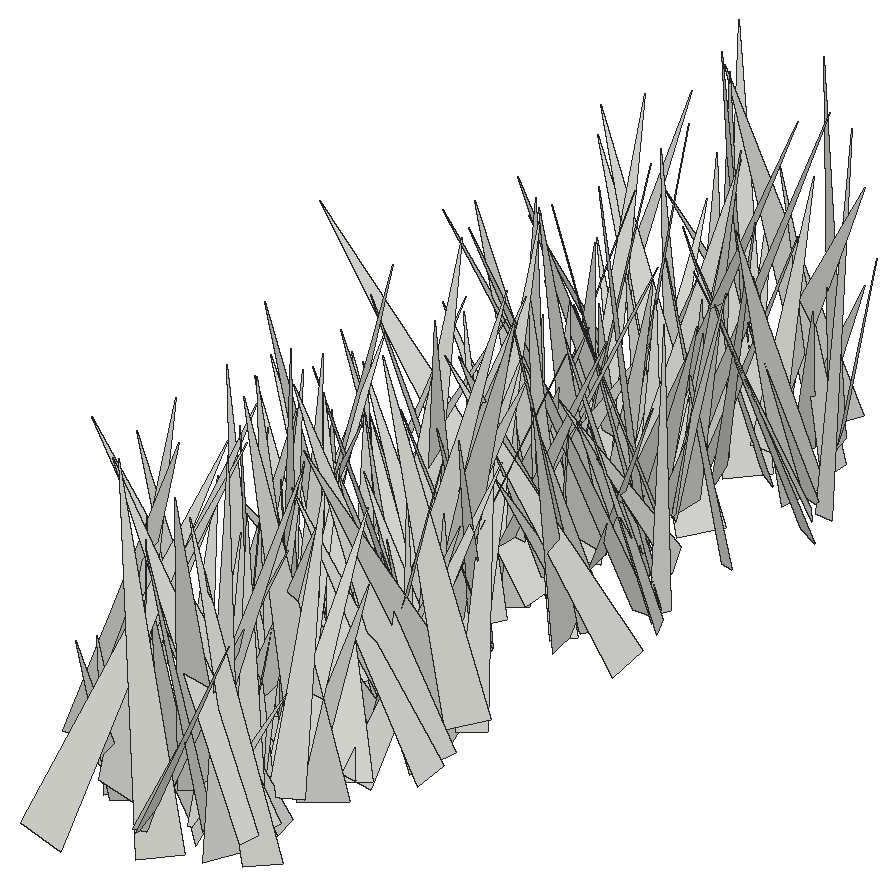
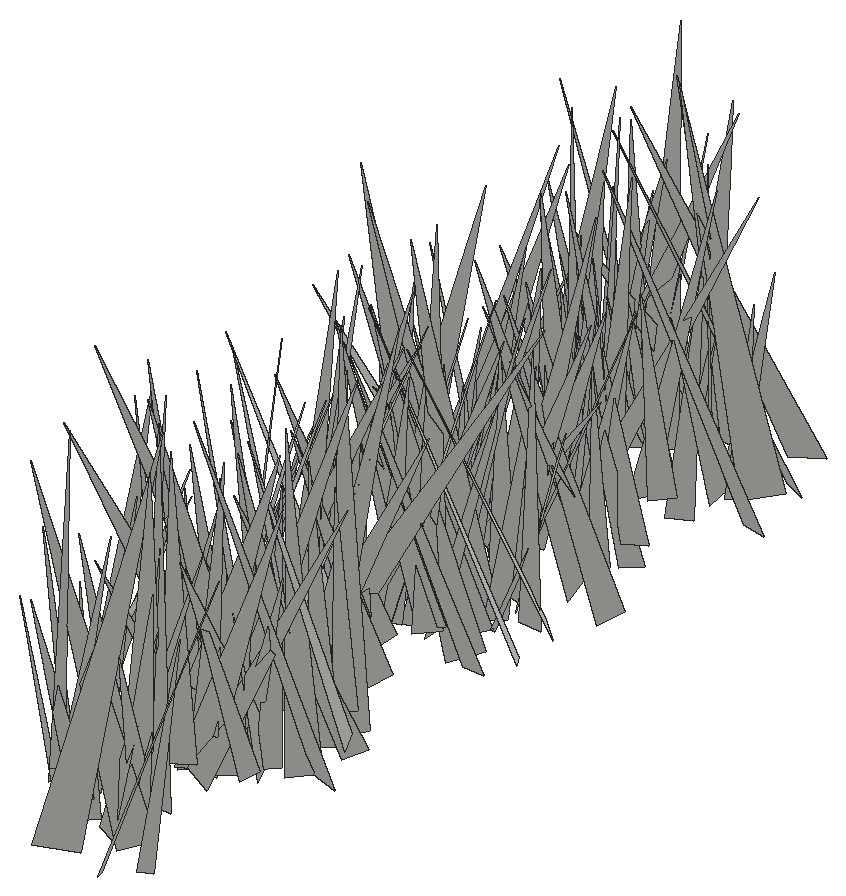
# SketchUp Ruby script. Lengths in inches.
U = 1.inch
M = Sketchup.active_model
def pt(a) = Geom::Point3d.new(a.map { |v| v * U })
def face(e, loops, mat)
  f = e.add_face(loops[0].map { |a| pt(a) })
  loops[1..].each { |l| e.add_face(l.map { |a| pt(a) }).erase! }
  f.material = f.back_material = mat if mat
  f
end
# faces: each face lists its corners as indices into pts; further lists are holes
def faces(e, pts, list, mat = nil) = list.each { |f| face(e, (f[0].is_a?(Array) ? f : [f]).map { |l| l.map { |i| pts[i] } }, mat) }
# xy, xz, yz: faces in a plane at the given z, y or x. An outline is a flat list of corners, or four numbers for a rectangle; further outlines are holes
def ring(l) = l.size == 4 ? [[l[0], l[1]], [l[2], l[1]], [l[2], l[3]], [l[0], l[3]]] : l.each_slice(2).to_a
def flat(e, list, mat, &to3) = list.each { |f| face(e, (f[0].is_a?(Array) ? f : [f]).map { |l| ring(l).map { |u, v| to3.(u, v) } }, mat) }
def xy(e, z, list, mat = nil) = flat(e, list, mat) { |x, y| [x, y, z] }
def xz(e, y, list, mat = nil) = flat(e, list, mat) { |x, z| [x, y, z] }
def yz(e, x, list, mat = nil) = flat(e, list, mat) { |y, z| [x, y, z] }
def lines(e, pts, list) = list.each { |a, b| e.add_line(pt(pts[a]), pt(pts[b])) }
# prism: a flat outline (further loops are holes) pulled along v
def prism(e, loops, v, mat = nil)
  f = face(e, loops, mat); d = Geom::Vector3d.new(v.map { |x| x * U })
  f.pushpull(f.normal.samedirection?(d) ? d.length : -d.length)
end
def box(e, o, s, mat = nil) = prism(e, [[o, [o[0] + s[0], o[1], o[2]], [o[0] + s[0], o[1] + s[1], o[2]], [o[0], o[1] + s[1], o[2]]]], [0, 0, s[2]], mat)
def at(x, y, z, deg = 0) = Geom::Transformation.translation(pt([x, y, z])) * Geom::Transformation.rotation(ORIGIN, Z_AXIS, deg.degrees)
def axes(o, x, y, z) = Geom::Transformation.new([*x, 0, *y, 0, *z, 0, *pt(o).to_a, 1])
def part(name) = M.definitions.add(name)
# library, detail: a bought-in or finely detailed component or shape, given as its bounding box
def library(name, o, s) = part(name).tap { |d| box(d.entities, o, s) }
def detail(e, o, s) = box(e.add_group.entities, o, s)
def put(e, d, t, mat = nil) = e.add_instance(d, t).tap { |i| i.material = mat if mat }
def group(e, t, mat = nil) = e.add_group.tap { |g| g.transformation = t; g.material = mat if mat }.entities
root = M.entities
c1 = part("fur_instance\#9")
p = [[0.8125,0,1.79],[0.67,-0.02,1.48],[0,-0.11,0],[0,0.11,0]]
faces(c1.entities,p,[[0,1,2,3]])
put(root,c1,axes([151.81,72.7,-28.22],[-5.03128,5.10175,2.45438],[5.52933,5.13327,0.66454],[1.21582,-2.23324,7.13442]))
put(root,c1,axes([151.36,72.26,-27.1],[3.9948,0.59542,0.26899],[0.55235,-3.96784,0.58004],[-0.34899,0.53573,3.99706]))
put(root,c1,axes([152.68,74.1,-27.1],[-4.88015,-2.78524,1.52655],[-2.68194,5.11285,0.7548],[1.7015,0.07051,5.5681]))
put(root,c1,axes([151.31,75.63,-27.1],[4.3126,-6.65441,0.44802],[-6.65528,-4.32849,-0.22777],[-0.435,0.25174,7.9264]))
put(root,c1,axes([148.35,74.96,-28.22],[1.6071,-3.85332,0.26864],[-3.82652,-1.62792,-0.45895],[-0.52725,0.06941,4.14972]))
put(root,c1,axes([147.79,71.21,-28.22],[0.28527,8.21503,1.11931],[7.94931,0.04717,-2.37217],[2.35543,-1.15413,7.87026]))
put(root,c1,axes([154.69,74.52,-27.1],[-6.88709,2.46248,0.81316],[2.58785,6.67518,1.70354],[0.16756,-1.88022,7.11293]))
put(root,c1,axes([151.44,73.41,-28.22],[1.87721,3.55983,2.07479],[3.45548,-2.60202,1.33802],[-2.2443,-1.02868,3.79553]))
put(root,c1,axes([149.46,74.71,-27.1],[4.52719,2.71843,2.25301],[3.1828,-4.72799,-0.69084],[-1.52829,-1.79378,5.23527]))
put(root,c1,axes([147.89,75.2,-28.22],[2.32734,-2.83374,0.7234],[-2.82694,-2.41664,-0.37171],[-0.74954,0.31569,3.64807]))
put(root,c1,axes([154.875,74.43,-28.22],[1.40362,-5.52471,3.15038],[-5.88186,-2.35471,-1.50878],[-2.41887,2.51999,5.49692]))
put(root,c1,axes([149.01,73.77,-27.1],[1.36969,7.27883,2.41401],[7.66649,-1.2409,-0.6083],[0.18385,-2.48268,7.38156]))
put(root,c1,axes([146.77,74.74,-27.1],[4.56446,-0.76979,0.5853],[-0.81155,-4.58493,0.29877],[-0.52586,0.39409,4.61927]))
put(root,c1,axes([153.43,73.97,-28.22],[-6.82221,1.72842,2.33339],[1.55801,7.20655,-0.7829],[2.45045,0.23004,6.99407]))
put(root,c1,axes([146,76,-27.1],[4.04324,-6.81137,0.9787],[-6.74817,-3.70246,2.11055],[1.34718,1.89668,7.63467]))
put(root,c1,axes([151.84,74.47,-28.22],[2.36408,2.77163,0.06713],[2.67068,-2.25294,-1.03299],[0.74428,-0.71945,3.49339]))
put(root,c1,axes([151.41,72.19,-27.1],[5.35308,0.77922,1.1136],[0.09871,-4.73607,2.83947],[-1.35556,2.73224,4.60435]))
put(root,c1,axes([146.69,73.35,-28.22],[4.52009,6.67395,0.30614],[6.59904,-4.40227,-1.46264],[1.04307,-1.07006,7.92676]))
put(root,c1,axes([152.66,76.88,-28.22],[-1.08369,-5.40972,1.03151],[-5.49173,1.14023,0.21038],[0.41232,0.96864,5.51318]))
put(root,c1,axes([153.82,76.95,-28.22],[-3.71284,-0.24914,0.82183],[0.046,3.58403,1.29433],[0.85753,-1.27095,3.48884]))
put(root,c1,axes([148.58,77.6,-28.22],[2.00782,-4.43373,0.05819],[-4.43409,-2.00742,0.0429],[0.01508,0.0707,4.86698]))
put(root,c1,axes([150.21,75.92,-28.22],[4.58596,6.39713,1.96066],[6.63658,-4.04695,-2.31874],[0.85046,-2.91504,7.52182]))
put(root,c1,axes([151.92,76.79,-27.1],[-3.79405,-1.81524,0.00607],[-1.81515,3.79397,0.03081],[0.01877,-0.02517,4.20582]))
put(root,c1,axes([153.38,75.6,-27.1],[-1.15441,5.11883,1.74969],[5.40957,1.09949,0.35248],[0.0216,-1.78472,5.23554]))
put(root,c1,axes([151.71,75,-28.22],[0.07202,5.27236,0.64208],[5.29211,-0.12578,0.43929],[-0.45123,-0.63374,5.25452]))
put(root,c1,axes([148.45,75.49,-28.22],[-4.01234,0.85775,1.7856],[0.34464,4.27421,-1.27879],[1.95072,1.00913,3.89863]))
put(root,c1,axes([151.82,75.75,-27.1],[1.21689,3.56799,0.58582],[3.55761,-1.29191,0.47847],[-0.64586,-0.39367,3.73931]))
put(root,c1,axes([152.39,77.26,-27.1],[-4.17203,-5.0841,2.64194],[-5.48144,4.49304,-0.00972],[1.66784,2.04897,6.57676]))
put(root,c1,axes([151.5,78.52,-27.1],[-6.98354,0.71492,0.27676],[0.75932,6.7998,1.59491],[0.10557,-1.6153,6.83646]))
put(root,c1,axes([149.4,78.76,-27.1],[-6.05597,0.77226,2.0179],[1.21073,6.18666,1.26588],[1.78953,-1.57224,5.97233]))
put(root,c1,axes([145.97,76.56,-28.22],[3.571,6.90444,0.98118],[6.89309,-3.32732,-1.67343],[1.05801,-1.62595,7.59098]))
put(root,c1,axes([153.72,79.16,-28.22],[2.92408,-7.38877,2.72238],[-7.56214,-3.44459,-1.22649],[-2.19528,2.02396,7.85111]))
put(root,c1,axes([153.84,77,-27.1],[3.74309,-3.05687,3.19875],[-4.02453,-4.09315,0.7978],[-1.83838,2.73658,4.76642]))
put(root,c1,axes([150.07,79.39,-27.1],[2.36521,-5.47601,0.71506],[-5.30162,-2.03369,1.96193],[1.54624,1.40343,5.6331]))
put(root,c1,axes([151.96,77.6875,-28.22],[-7.50799,1.69583,1.59774],[1.55933,7.66276,-0.80567],[1.73121,0.45255,7.65484]))
put(root,c1,axes([150.21,79.22,-28.22],[3.90059,1.73334,0.99556],[1.91928,-3.85762,-0.80331],[-0.55855,-1.15086,4.19211]))
put(root,c1,axes([148.73,78.4,-27.1],[-3.00951,3.51493,1.30262],[3.55292,3.20728,-0.44587],[1.1951,-0.68362,4.60577]))
put(root,c1,axes([153.36,77.51,-27.1],[-2.46279,4.53865,0.90199],[4.34757,2.61941,-1.3098],[1.58479,-0.13272,4.99491]))
put(root,c1,axes([151.4375,78.15,-28.22],[1.82838,5.64567,1.15342],[5.69001,-1.95997,0.57384],[-0.90985,-0.91206,5.90655]))
put(root,c1,axes([152.03,79.75,-28.22],[-4.40906,-3.22075,2.19411],[-3.50304,4.72714,-0.10035],[1.70765,1.38134,5.45921]))
put(root,c1,axes([152.3,80.49,-27.1],[2.6099,-2.39325,0.8726],[-2.54736,-2.4537,0.88934],[-0.00348,1.24593,3.42758]))
put(root,c1,axes([150.16,81.75,-27.1],[7.38345,1.68053,2.79244],[2.22073,-7.65548,-1.26461],[-2.38543,-1.92527,7.46594]))
put(root,c1,axes([149.39,80.07,-27.1],[-4.16278,-2.64249,2.71758],[-3.23685,4.57857,-0.50613],[1.97251,1.93665,4.90462]))
put(root,c1,axes([152.11,78.94,-28.22],[-3.17134,4.85922,0.78552],[4.77597,3.26378,-0.90795],[1.19131,-0.14895,5.73106]))
put(root,c1,axes([150.39,81.34,-27.1],[1.19646,-6.35488,2.45253],[-6.76034,-1.41301,-0.36331],[-0.83491,2.33448,6.45631]))
put(root,c1,axes([152.5,79.18,-28.22],[-7.20595,2.28011,2.02761],[1.9171,7.42879,-1.54068],[2.37378,0.922,7.39939]))
put(root,c1,axes([147.42,81.61,-27.1],[0.1838,-6.38239,2.38865],[-6.46729,0.58989,2.0738],[2.14821,2.32195,6.03888]))
put(root,c1,axes([149.875,82,-28.22],[-4.52682,2.09063,1.69581],[2.46981,4.54531,0.98938],[1.07078,-1.64562,4.88712]))
put(root,c1,axes([147.71,81.42,-28.22],[1.71183,-4.04593,1.56999],[-4.29437,-1.33542,1.2409],[0.62675,1.9005,4.21427]))
put(root,c1,axes([155.48,82.79,-28.22],[-5.93019,0.58333,0.46706],[0.68124,5.75556,1.46115],[0.30714,-1.50292,5.77689]))
put(root,c1,axes([154.98,83.53,-28.22],[-6.87965,3.10007,2.46286],[3.78941,6.58637,2.29475],[1.14737,-3.16466,7.18848]))
put(root,c1,axes([153.61,80.83,-28.22],[-2.77056,6.19265,0.76015],[6.19361,2.62958,1.15202],[-0.75223,-1.15721,6.68563]))
put(root,c1,axes([150,81.97,-27.1],[-4.89428,-1.48699,1.50253],[-1.73277,4.99254,-0.70337],[1.21087,1.13406,5.0666]))
put(root,c1,axes([154.04,86.47,-28.22],[-7.59167,-1.95799,2.55179],[-0.44126,7.11339,4.14535],[3.18601,-3.68034,6.65457]))
put(root,c1,axes([151.45,84.84,-28.22],[-4.13984,-2.04423,0.54277],[-1.65039,3.86825,1.98107],[1.32277,-1.57147,4.17043]))
put(root,c1,axes([147.37,83.73,-27.1],[0.94706,-3.59902,0.23008],[-3.53322,-0.8783,0.80484],[0.72266,0.42244,3.63347]))
put(root,c1,axes([150.06,81.22,-27.1],[-5.67085,1.89535,1.35099],[1.57668,5.74544,-1.44226],[1.71219,0.98676,5.80265]))
put(root,c1,axes([151.85,82.4375,-28.22],[-3.49983,5.63032,0.78088],[5.54982,3.18646,1.89866],[-1.22869,-1.64469,6.35172]))
put(root,c1,axes([153.53,84.65,-27.1],[-0.97443,-3.66118,0.75209],[-3.71136,1.03977,0.25308],[0.44234,0.6588,3.78017]))
put(root,c1,axes([151.94,83.9375,-28.22],[5.73054,2.09287,1.0832],[2.24178,-5.71944,-0.8093],[-0.7265,-1.14039,6.04684]))
put(root,c1,axes([151.41,86.41,-27.1],[5.27025,-2.47106,0.85487],[-2.00329,-5.05203,-2.25305],[-1.68041,-1.72721,5.36707]))
put(root,c1,axes([155.46,84.81,-27.1],[3.76435,-5.16952,3.38659],[-5.24976,-4.76711,-1.44149],[-3.26082,1.70703,6.23028]))
put(root,c1,axes([148.71,88.21,-28.22],[-5.34969,-3.46152,0.37635],[-2.75195,4.62606,3.43064],[2.1332,-2.713,5.36954]))
put(root,c1,axes([151.6875,84.97,-27.1],[-1.12844,-4.06047,0.83548],[-3.60524,0.5338,-2.27512],[-2.04639,1.29864,3.54749]))
put(root,c1,axes([149.98,85.82,-28.22],[-1.48143,-7.59825,2.03928],[-7.84224,1.26126,-0.99758],[-0.62555,2.18232,7.67677]))
put(root,c1,axes([145.93,84.86,-28.22],[6.32443,-0.86949,0.03215],[-0.87008,-6.31952,0.24926],[0.00213,0.25131,6.37905]))
put(root,c1,axes([153.91,83.67,-28.22],[0.68638,4.30492,0.85677],[4.11958,-0.93113,1.37825],[-1.51508,-0.58153,4.13569]))
put(root,c1,axes([153.75,80.92,-28.22],[-5.06896,3.36354,0.19703],[2.56301,4.08037,-3.71862],[2.18706,3.01393,4.81452]))
put(root,c1,axes([151.89,85.47,-27.1],[0.78956,-4.05986,1.16414],[-3.93825,-0.27989,1.69498],[1.52574,1.37851,3.77266]))
put(root,c1,axes([150.81,84.85,-27.1],[-4.45803,3.98436,0.74293],[4.03358,4.25341,1.39275],[-0.39655,-1.52789,5.81458]))
put(root,c1,axes([152.47,86.12,-28.22],[2.98723,-2.64764,1.00912],[-2.72025,-3.09017,-0.05514],[-0.79284,0.62671,3.99131]))
put(root,c1,axes([153.46,85.88,-27.1],[-3.79672,1.89832,0.59417],[1.98792,3.66583,0.99077],[0.06937,-1.15319,4.1276]))
put(root,c1,axes([147.94,83.45,-27.1],[0.187,6.43803,0.46404],[6.40843,-0.12967,-0.78342],[0.77175,-0.48321,6.39292]))
put(root,c1,axes([152.16,87.03,-28.22],[-3.80657,-5.75041,0.9295],[-5.82495,3.76407,-0.56819],[0.03325,1.08891,6.87272]))
put(root,c1,axes([152,85.7,-27.1],[-4.7779,-0.84592,1.0787],[-0.97294,4.84801,-0.50762],[0.9657,0.69908,4.82558]))
put(root,c1,axes([148.35,83.6,-28.22],[-7.17026,0.40545,3.85637],[-0.86926,7.73252,-2.42922],[3.77894,2.54801,6.75839]))
put(root,c1,axes([149.12,87.5,-28.22],[4.28198,-1.79299,1.3249],[-1.43721,-4.41332,-1.32759],[-1.70429,-0.78312,4.44833]))
put(root,c1,axes([149.2,86.18,-28.22],[-3.51582,-2.14374,0.80605],[-2.26912,3.46073,-0.69338],[0.31056,1.01688,4.05904]))
put(root,c1,axes([152.64,86.91,-27.1],[1.6475,-3.20979,0.84583],[-3.31321,-1.64761,0.20101],[-0.20196,0.8456,3.6023]))
put(root,c1,axes([147.85,87.13,-28.22],[-0.76363,-5.08076,1.72351],[-5.30047,0.98391,0.55201],[0.83046,1.60796,5.10809]))
put(root,c1,axes([150.55,85.31,-28.22],[-5.6137,1.8249,1.28834],[1.63706,5.7317,-0.98561],[1.51991,0.56669,5.82001]))
put(root,c1,axes([151.17,86.39,-27.1],[1.96643,7.28816,1.86053],[7.47956,-1.69089,-1.28167],[0.79683,-2.11408,7.43918]))
put(root,c1,axes([152.9,87.72,-28.22],[-5.49496,2.98551,0.84144],[3.09795,5.36781,1.18541],[0.15494,-1.44541,6.14025]))
put(root,c1,axes([151.63,87.08,-27.1],[-3.45745,4.3845,0.64107],[4.38114,3.2607,1.32749],[-0.66366,-1.31634,5.42361]))
put(root,c1,axes([152.15,89.65,-27.1],[-0.85203,-5.57664,0.61964],[-5.3803,0.98986,1.51043],[1.59225,0.36067,5.43539]))
put(root,c1,axes([150.91,88.7,-27.1],[6.79044,-4.4332,0.71146],[-4.48312,-6.76549,0.63187],[-0.24718,0.91888,8.0848]))
put(root,c1,axes([152.17,85.34,-27.1],[5.76242,3.50846,0.12226],[3.39302,-5.62636,1.53663],[-0.90093,1.2508,6.56914]))
put(root,c1,axes([151.55,88.95,-28.22],[0.38747,-3.62863,0.53891],[-3.66751,-0.39531,-0.02484],[-0.08219,0.53319,3.64917]))
put(root,c1,axes([154.625,86.09,-28.22],[-5.36407,2.31527,0.60969],[2.0889,5.25672,-1.5839],[1.1699,1.22955,5.6236]))
put(root,c1,axes([152.35,90.04,-27.1],[-3.97091,-3.72473,0.66515],[-3.58252,4.01146,1.07602],[1.21718,-0.34456,5.33703]))
put(root,c1,axes([149.09,88.69,-28.22],[1.67696,-6.87357,2.26471],[-6.67493,-0.57073,3.21041],[2.79647,2.7596,6.30488]))
put(root,c1,axes([150.25,89.63,-28.22],[-6.39849,-1.36399,1.46981],[-1.16574,6.52941,0.98452],[1.63152,-0.68393,6.46776]))
put(root,c1,axes([150.28,87.375,-28.22],[-4.94866,6.16749,2.69055],[6.18584,5.48419,-1.19385],[2.6481,-1.28527,7.81677]))
put(root,c1,axes([149.18,91.26,-27.1],[7.15666,-2.1147,0.99823],[-1.83229,-7.06792,-1.83669],[-1.45298,-1.50292,7.233]))
put(root,c1,axes([150.68,91.56,-27.1],[-1.15105,-5.30671,0.17],[-5.09537,1.15297,1.49093],[1.49242,-0.15644,5.22142]))
put(root,c1,axes([147.22,86.81,-28.22],[4.61833,5.37447,0.17353],[5.34108,-4.61135,0.67253],[-0.62281,0.30742,7.05419]))
put(root,c1,axes([150.89,91.33,-27.1],[-5.52316,-3.7636,0.965],[-3.71814,5.60658,0.58551],[1.12752,0.05244,6.65787]))
put(root,c1,axes([151.23,89.73,-28.22],[-2.08975,2.94897,0.92989],[3.09202,1.98432,0.65582],[-0.0238,-1.13764,3.55435]))
put(root,c1,axes([148.27,90.33,-28.22],[5.35038,-4.23141,0.69897],[-4.27634,-5.17862,1.38378],[0.32603,1.51562,6.67957]))
put(root,c1,axes([145.36,90.97,-27.1],[5.77692,4.11347,0.10405],[3.90568,-5.42514,-2.37018],[1.29504,-1.98782,6.68399]))
put(root,c1,axes([153.22,92.94,-28.22],[5.83634,-0.86723,1.56304],[-0.35494,-5.79341,-1.88904],[-1.75191,-1.71533,5.58985]))
put(root,c1,axes([155.84,93.03,-28.22],[-6.77007,0.71674,0.61078],[0.8862,6.3486,2.37288],[0.31848,-2.42944,6.38099]))
put(root,c1,axes([152.09,94.48,-27.1],[4.15216,-5.25606,0.30062],[-4.95254,-4.0295,-2.04756],[-1.78575,-1.04593,6.37763]))
put(root,c1,axes([151.65,90.79,-27.1],[-4.9618,2.41645,1.1014],[2.44275,5.06865,-0.11597],[1.04177,-0.37582,5.51772]))
put(root,c1,axes([149.36,90.95,-27.1],[-0.86303,4.80618,1.97762],[4.83833,1.47497,-1.47315],[1.8976,-1.57489,4.65553]))
put(root,c1,axes([152.28,88.4,-28.22],[0.71123,8.26754,0.30404],[8.18462,-0.74766,1.1847],[-1.20692,-0.19821,8.21307]))
put(root,c1,axes([152.4375,94.43,-27.1],[-3.66849,-5.82093,1.22872],[-5.44278,3.86666,2.06783],[2.40191,-0.1285,6.56241]))
put(root,c1,axes([147.4,90.95,-28.22],[2.61038,6.20008,1.07332],[6.21386,-2.35716,-1.49626],[0.99041,-1.55238,6.55868]))
put(root,c1,axes([153.51,94.07,-28.22],[1.73038,-3.85975,0.19684],[-3.59553,-1.68683,-1.46882],[-1.41726,-0.43309,3.96667]))
put(root,c1,axes([151.82,93.66,-27.1],[-7.78216,2.50032,0.23977],[2.4235,7.26917,2.85602],[-0.66011,-2.78901,7.65877]))
put(root,c1,axes([150.41,93.71,-28.22],[2.93376,-3.22318,1.07266],[-3.3076,-3.03341,-0.06853],[-0.77414,0.74566,4.35788]))
put(root,c1,axes([149.96,92.89,-27.1],[5.54197,-0.978,0.47716],[-1.05474,-5.437,1.10644],[-0.26776,1.17482,5.51777]))
put(root,c1,axes([152.16,94.625,-28.22],[-4.33976,4.07233,1.17149],[4.17045,3.80756,2.21352],[-0.75076,-2.38923,5.52429]))
put(root,c1,axes([151.52,96.08,-28.22],[4.21418,-1.38432,0.79636],[-0.98829,-4.02576,-1.76817],[-1.25452,-1.47878,4.06808]))
put(root,c1,axes([151.81,94.16,-28.22],[-2.43911,-2.15453,1.73505],[-2.51562,2.68975,-0.19638],[1.15067,1.31336,3.24849]))
put(root,c1,axes([153.06,93.04,-28.22],[-1.53438,4.71255,0.03454],[4.47921,1.44703,1.55125],[-1.46492,-0.51147,4.70702]))
put(root,c1,axes([150.33,95.79,-28.22],[0.4786,-6.17329,1.68247],[-6.39725,-0.42884,0.2463],[0.12453,1.69584,6.18692]))
put(root,c1,axes([154.1,96.13,-28.22],[-3.30387,-7.05223,0.96215],[-6.92829,2.9435,-2.21582],[-1.63048,1.78244,7.4659]))
put(root,c1,axes([154.47,96.24,-28.22],[-3.61548,-1.81279,0.7212],[-1.71327,3.67656,0.65243],[0.9333,-0.2734,3.99152]))
put(root,c1,axes([150.83,97.14,-27.1],[-0.69616,-7.71222,1.47846],[-7.81205,0.83092,0.65597],[0.79755,1.40715,7.71575]))
put(root,c1,axes([152.71,97.56,-27.1],[3.43107,-2.8474,0.0502],[-2.64084,-3.2106,-1.6126],[-1.06592,-1.21113,4.15686]))
put(root,c1,axes([153.89,98.12,-27.1],[-4.54437,-2.07997,0.71062],[-1.49312,4.11891,2.50752],[1.61302,-2.04715,4.32318]))
put(root,c1,axes([155.09,95.73,-28.22],[-5.70122,-3.26457,0.62497],[-3.32356,5.6155,-0.98593],[0.04408,1.16649,6.49533]))
put(root,c1,axes([149.75,96.99,-27.1],[-6.14349,2.42883,3.06477],[3.31416,6.26335,1.67969],[2.07568,-2.81172,6.38908]))
put(root,c1,axes([151.89,96.27,-27.1],[4.55769,0.07164,0.01251],[0.0727,-4.46545,-0.91231],[0.00209,-0.91239,4.46602]))
put(root,c1,axes([148.31,95.18,-27.1],[4.95013,-1.23925,0.4471],[-1.29852,-4.88303,0.8422],[-0.22245,0.9272,5.03291]))
put(root,c1,axes([148.92,95.44,-27.1],[6.16739,3.42449,0.19717],[3.4017,-6.05394,-1.25736],[0.441,-1.19388,6.94138]))
put(root,c1,axes([151.17,99.13,-28.22],[-6.65977,-5.09555,0.25994],[-4.96209,6.56797,1.61994],[1.1874,-1.13219,8.22757]))
put(root,c1,axes([147.93,97.44,-28.22],[7.26083,-2.43104,1.92439],[-2.31077,-7.51014,-0.76873],[-2.06726,-0.14373,7.61831]))
put(root,c1,axes([152.8,99.03,-27.1],[-3.72414,-4.2026,0.59605],[-4.10843,3.76818,0.89886],[1.06672,-0.15915,5.54285]))
put(root,c1,axes([154.18,96.96,-28.22],[-6.0406,-4.0795,1.11122],[-4.22494,5.74856,-1.86274],[-0.16426,2.16279,7.04708]))
put(root,c1,axes([147.875,97.79,-27.1],[-2.80028,2.24736,2.49663],[2.73085,3.4158,-0.01176],[1.95607,-1.55147,3.59055]))
put(root,c1,axes([154.5,96.5,-28.22],[-4.924,0.48292,1.1816],[0.20052,4.94285,-1.18453],[1.26062,1.10005,4.80373]))
put(root,c1,axes([152.61,98.18,-28.22],[-6.29622,-3.82649,2.40942],[-4.00808,6.63484,0.06324],[2.09347,1.19444,7.36752]))
put(root,c1,axes([148.12,98.65,-28.22],[2.86346,-4.49186,1.0378],[-4.60706,-2.8331,0.44926],[-0.16992,1.11803,5.30796]))
put(root,c1,axes([150.3,99.11,-27.1],[-0.32261,-5.78503,1.74562],[-5.69921,0.87225,1.8374],[2.00818,1.5461,5.49497]))
put(root,c1,axes([150.92,100.06,-27.1],[-1.61608,-6.86234,1.14057],[-6.89566,1.42577,-1.19223],[-0.91789,1.37106,6.94853]))
put(root,c1,axes([146.88,98.43,-28.22],[2.54302,-4.52945,1.06711],[-4.23804,-1.75205,2.66287],[1.92189,2.12978,4.46004]))
put(root,c1,axes([148.28,99.0625,-28.22],[7.04246,3.4796,1.7186],[3.70112,-7.09298,-0.80545],[-1.16744,-1.49647,7.81378]))
put(root,c1,axes([147.36,100.79,-28.22],[5.23742,-3.794,0.7561],[-3.79638,-5.28528,-0.22367],[-0.74406,0.26094,6.46336]))
put(root,c1,axes([150.54,100.74,-28.22],[5.31861,-1.95589,0.12332],[-1.94358,-5.30997,-0.39374],[-0.25139,-0.32717,5.65315]))
put(root,c1,axes([148.67,101.18,-28.22],[4.83805,-1.95602,0.87332],[-1.75837,-4.85831,-1.14034],[-1.22345,-0.75248,5.09238]))
put(root,c1,axes([146.38,99.43,-27.1],[5.52496,2.9641,0.73245],[3.00682,-5.54515,-0.24054],[-0.53047,-0.55942,6.26523]))
put(root,c1,axes([151.6,100.73,-27.1],[3.4231,3.63538,1.50249],[3.93251,-3.11512,-1.42212],[0.09387,-2.06666,4.78656]))
put(root,c1,axes([150.12,97.65,-28.22],[0.0768,8.17284,0.16546],[8.06568,-0.10268,1.32775],[-1.3295,-0.15078,8.06464]))
put(root,c1,axes([154.24,100.41,-28.22],[-3.42492,-4.02626,1.68032],[-4.34426,2.9504,-1.78518],[-0.40205,2.41841,4.97534]))
put(root,c1,axes([150.51,100.83,-28.22],[-2.37433,3.47563,1.70417],[3.72029,2.6012,-0.12184],[1.06942,-1.33243,4.20745]))
put(root,c1,axes([150.6,99.37,-27.1],[8.13769,0.92636,1.08085],[0.65484,-8.00564,1.93114],[-1.26395,1.81658,7.95932]))
put(root,c1,axes([151.89,101.11,-27.1],[7.00703,0.38351,2.14023],[0.30488,-7.32356,0.31416],[-2.15283,0.21111,7.01048]))
put(root,c1,axes([150.28,100.3,-28.22],[-1.59502,6.99566,2.35908],[7.02793,2.17795,-1.70682],[2.26111,-1.83463,6.96922]))
put(root,c1,axes([148.68,101.51,-28.22],[7.03431,3.48518,2.0857],[3.73576,-7.18871,-0.58711],[-1.59396,-1.46769,7.82836]))
put(root,c1,axes([150.22,103.36,-28.22],[-2.23247,-5.83337,0.18602],[-5.6892,2.13065,-1.46288],[-1.30221,0.692,6.07224]))
put(root,c1,axes([149.88,100.78,-27.1],[-3.84574,2.31871,0.01808],[2.31862,3.84577,-0.02193],[0.02681,0.00945,4.49062]))
put(root,c1,axes([150.82,102.86,-28.22],[4.27597,-2.96302,0.67606],[-2.94629,-4.32773,-0.33261],[-0.74558,0.10858,5.19161]))
put(root,c1,axes([149.53,102.44,-28.22],[-3.6167,2.28369,2.19841],[2.80718,3.85669,0.61192],[1.47241,-1.74341,4.23336]))
put(root,c1,axes([152.1,101.7,-28.22],[-4.97351,5.86998,1.15657],[5.9442,4.67754,1.82131],[-0.6788,-2.04794,7.47498]))
put(root,c1,axes([151.5,103.375,-27.1],[6.22131,1.299,1.34326],[1.60809,-6.10017,-1.54868],[-0.95174,-1.81575,6.1639]))
put(root,c1,axes([155.07,103.76,-28.22],[-2.96525,-5.05492,0.58848],[-5.08807,2.93137,-0.45808],[-0.10025,0.73898,5.84252]))
put(root,c1,axes([146.51,100.7,-28.22],[3.51205,7.24819,1.1392],[7.33442,-3.43356,-0.76524],[0.20101,-1.35755,8.01781]))
put(root,c1,axes([155.51,103.42,-27.1],[-3.79986,-3.34827,0.10157],[-3.34083,3.7767,-0.4853],[-0.24505,0.43103,5.04126]))
put(root,c1,axes([150.25,100.12,-28.22],[-4.13598,4.27474,0.09369],[4.07434,3.97972,-1.71759],[1.29691,1.13001,5.6947]))
put(root,c1,axes([150.52,102.65,-28.22],[-1.16984,-6.03511,2.92768],[-6.70455,0.96018,-0.69968],[-0.2073,3.00298,6.1075]))
put(root,c1,axes([153.25,105.83,-28.22],[6.17469,-3.94346,0.96595],[-3.5616,-6.10514,-2.15707],[-1.94909,-1.33681,7.00177]))
put(root,c1,axes([150.74,102.83,-28.22],[-5.22041,4.31379,0.87725],[4.39805,5.05275,1.32586],[-0.18846,-1.57859,6.64105]))
put(root,c1,axes([151.63,100.25,-27.1],[7.3603,1.92647,1.4977],[1.22652,-7.03518,3.02165],[-2.10951,2.63124,6.98247]))
put(root,c1,axes([147.59,103.6,-27.1],[4.04534,-0.8517,0.30361],[-0.87788,-4.03293,0.38361],[-0.21657,0.43867,4.11619]))
put(root,c1,axes([153.625,105.74,-28.22],[-0.76321,-4.71965,0.1503],[-4.6984,0.77422,0.45372],[0.47201,0.07524,4.75939]))
put(root,c1,axes([150.23,104.47,-27.1],[2.8988,-5.16102,2.16058],[-5.5292,-3.01461,0.21733],[-0.85564,1.9958,5.91539]))
put(root,c1,axes([151.37,102.31,-27.1],[4.47299,1.54799,0.88013],[1.09405,-4.26651,1.94385],[-1.40498,1.60599,4.31572]))
put(root,c1,axes([152.8,106.39,-28.22],[-0.50575,-5.47671,0.42869],[-5.44927,0.55465,0.65709],[0.69543,0.36321,5.46062]))
put(root,c1,axes([151.61,105.92,-28.22],[-2.91722,-4.26379,0.81225],[-4.33997,2.88016,-0.46811],[0.06569,0.93518,5.14499]))
put(root,c1,axes([149.46,107.54,-27.1],[-3.95013,-6.45103,2.53754],[-6.55598,4.42551,1.04517],[2.25256,1.56763,7.49179]))
put(root,c1,axes([148.78,107.46,-27.1],[-1.6159,-6.90986,2.38073],[-7.13771,2.01606,1.00679],[1.57067,2.05292,7.0245]))
put(root,c1,axes([151.37,108.13,-28.22],[4.03439,-1.67825,0.01541],[-1.64329,-3.95818,-0.85174],[-0.3411,-0.78061,4.28572]))
put(root,c1,axes([151.5,105.97,-27.1],[-0.63443,5.02312,1.44392],[5.17666,0.80438,-0.52377],[0.72032,-1.3566,5.03586]))
put(root,c1,axes([150.89,105.74,-28.22],[-6.71454,4.39928,1.56364],[4.39375,6.8803,-0.4901],[1.57912,-0.43767,8.0124]))
put(root,c1,axes([154.67,105.14,-28.22],[2.80201,6.02167,1.40008],[5.6342,-3.12002,2.14317],[-2.54489,-0.27744,6.28638]))
put(root,c1,axes([148.84,108.56,-28.22],[3.33833,-6.51025,0.54896],[-6.14625,-2.92038,2.74304],[2.21549,1.70799,6.78259]))
put(root,c1,axes([153,107.77,-28.22],[-5.71627,0.02456,1.51927],[0.09668,5.9079,0.26822],[1.51639,-0.28405,5.71003]))
put(root,c1,axes([153.32,107.5625,-27.1],[-6.66859,-2.01923,2.71074],[-2.32845,7.09045,-0.44648],[2.45024,1.24248,6.95328]))
put(root,c1,axes([150.27,108.56,-28.22],[-1.63509,-3.83691,0.93062],[-3.94815,1.58786,-0.39017],[-0.00453,1.00909,4.15248]))
put(root,c1,axes([147.37,109.91,-28.22],[-0.82646,-4.24361,0.01629],[-4.06802,0.79698,1.2278],[1.20816,-0.21938,4.14533]))
put(root,c1,axes([150.5,106.67,-28.22],[-4.40287,4.25609,0.42122],[4.26988,4.40886,0.08361],[0.24458,-0.35298,6.12311]))
put(root,c1,axes([150.99,110.54,-28.22],[5.28612,-6.00356,2.19792],[-5.60526,-5.72373,-2.15328],[-3.07484,0.113,7.70384]))
put(root,c1,axes([151.19,108.79,-27.1],[2.68666,-2.71893,0.01615],[-2.65256,-2.616,0.85524],[0.59729,0.61233,3.72549]))
put(root,c1,axes([148.58,111.03,-28.22],[-4.92711,-3.11526,0.5387],[-2.69685,4.66208,2.29422],[1.64986,-1.68274,5.3589]))
put(root,c1,axes([150.2,106.49,-28.22],[-4.43133,1.84787,0.51045],[1.62369,4.30117,-1.47494],[1.01922,1.18203,4.56901]))
put(root,c1,axes([153.03,108.09,-27.1],[3.30994,1.56111,0.94089],[1.62723,-3.40964,-0.0672],[-0.82125,-0.46405,3.659]))
